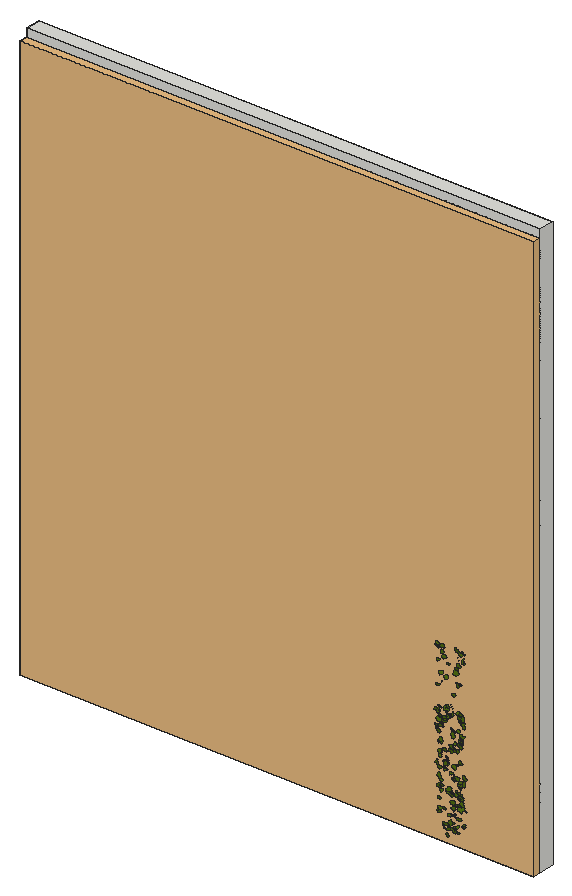
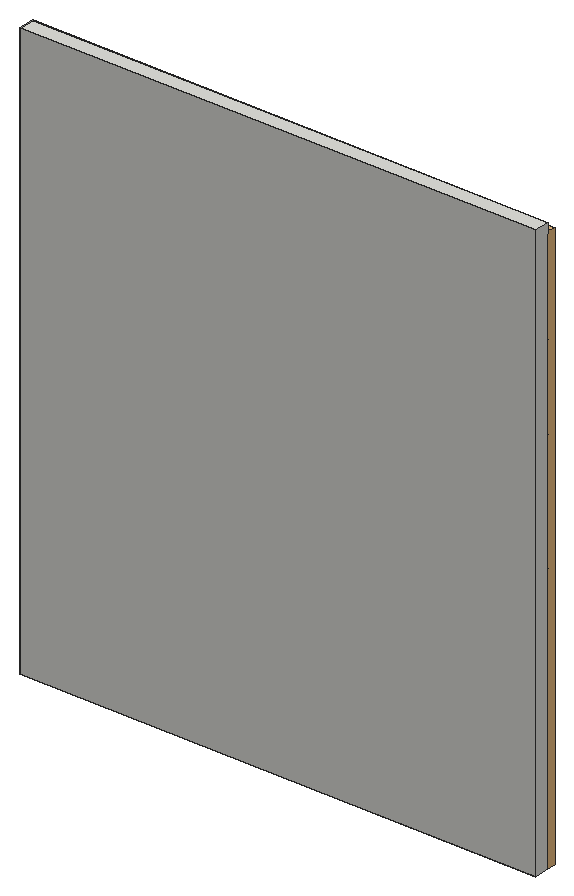
# SketchUp Ruby script. Lengths in inches.
U = 1.inch
M = Sketchup.active_model
def pt(a) = Geom::Point3d.new(a.map { |v| v * U })
def face(e, loops, mat)
  f = e.add_face(loops[0].map { |a| pt(a) })
  loops[1..].each { |l| e.add_face(l.map { |a| pt(a) }).erase! }
  f.material = f.back_material = mat if mat
  f
end
# faces: each face lists its corners as indices into pts; further lists are holes
def faces(e, pts, list, mat = nil) = list.each { |f| face(e, (f[0].is_a?(Array) ? f : [f]).map { |l| l.map { |i| pts[i] } }, mat) }
# xy, xz, yz: faces in a plane at the given z, y or x. An outline is a flat list of corners, or four numbers for a rectangle; further outlines are holes
def ring(l) = l.size == 4 ? [[l[0], l[1]], [l[2], l[1]], [l[2], l[3]], [l[0], l[3]]] : l.each_slice(2).to_a
def flat(e, list, mat, &to3) = list.each { |f| face(e, (f[0].is_a?(Array) ? f : [f]).map { |l| ring(l).map { |u, v| to3.(u, v) } }, mat) }
def xy(e, z, list, mat = nil) = flat(e, list, mat) { |x, y| [x, y, z] }
def xz(e, y, list, mat = nil) = flat(e, list, mat) { |x, z| [x, y, z] }
def yz(e, x, list, mat = nil) = flat(e, list, mat) { |y, z| [x, y, z] }
def lines(e, pts, list) = list.each { |a, b| e.add_line(pt(pts[a]), pt(pts[b])) }
# prism: a flat outline (further loops are holes) pulled along v
def prism(e, loops, v, mat = nil)
  f = face(e, loops, mat); d = Geom::Vector3d.new(v.map { |x| x * U })
  f.pushpull(f.normal.samedirection?(d) ? d.length : -d.length)
end
def box(e, o, s, mat = nil) = prism(e, [[o, [o[0] + s[0], o[1], o[2]], [o[0] + s[0], o[1] + s[1], o[2]], [o[0], o[1] + s[1], o[2]]]], [0, 0, s[2]], mat)
def at(x, y, z, deg = 0) = Geom::Transformation.translation(pt([x, y, z])) * Geom::Transformation.rotation(ORIGIN, Z_AXIS, deg.degrees)
def axes(o, x, y, z) = Geom::Transformation.new([*x, 0, *y, 0, *z, 0, *pt(o).to_a, 1])
def part(name) = M.definitions.add(name)
# library, detail: a bought-in or finely detailed component or shape, given as its bounding box
def library(name, o, s) = part(name).tap { |d| box(d.entities, o, s) }
def detail(e, o, s) = box(e.add_group.entities, o, s)
def put(e, d, t, mat = nil) = e.add_instance(d, t).tap { |i| i.material = mat if mat }
def group(e, t, mat = nil) = e.add_group.tap { |g| g.transformation = t; g.material = mat if mat }.entities
root = M.entities
M.materials.add("[Vegetation Blur 03]").color = [83, 114, 18]
c1 = library("Group\#9",[0,0,0],[130,2,144])
c2 = part("ivy")
xy(c2.entities,0,[[0.782,0,0.786,0,0.787,0.005,0.789,0.009,0.821,0.072,0.875,0.147,1.001,0.272,1.073,0.331,1.137,0.363,1.178,0.379,1.223,0.384,1.272,0.383,1.311,0.374,1.36,0.355,1.399,0.334,1.491,0.285,1.541,0.244,1.583,0.199,1.617,0.15,1.64,0.128,1.662,0.115,1.717,0.105,1.745,0.093,1.784,0.054,1.819,0.057,1.854,0.064,1.882,0.075,1.896,0.074,1.91,0.071,1.937,0.063,1.964,0.053,1.99,0.038,2.016,0.015,2.034,0.002,2.04,0,2.038,0.003,2.036,0.007,2.033,0.038,2.036,0.068,2.045,0.1,2.055,0.116,2.064,0.123,2.077,0.129,2.088,0.129,2.106,0.132,2.118,0.13,2.179,0.132,2.207,0.133,2.225,0.133,2.242,0.138,2.22,0.162,2.207,0.186,2.206,0.213,2.212,0.236,2.228,0.262,2.247,0.274,2.298,0.283,2.355,0.294,2.37,0.296,2.376,0.295,2.377,0.3,2.377,0.303,2.385,0.329,2.411,0.37,2.426,0.392,2.449,0.407,2.511,0.426,2.561,0.444,2.619,0.466,2.589,0.469,2.561,0.476,2.501,0.5,2.449,0.516,2.424,0.523,2.401,0.535,2.377,0.556,2.372,0.568,2.36,0.575,2.268,0.586,2.225,0.592,2.207,0.599,2.194,0.61,2.143,0.65,2.13,0.664,2.122,0.682,2.123,0.7,2.13,0.719,2.148,0.75,2.17,0.781,2.195,0.807,2.221,0.828,2.284,0.874,2.291,0.88,2.288,0.887,2.276,0.9,2.267,0.916,2.265,0.933,2.273,0.967,2.292,1.002,2.313,1.03,2.334,1.054,2.348,1.067,2.358,1.074,2.363,1.076,2.362,1.081,2.35,1.094,2.347,1.11,2.35,1.143,2.359,1.18,2.385,1.254,2.415,1.324,2.448,1.393,2.45,1.4,2.446,1.398,2.44,1.394,2.427,1.383,2.402,1.36,2.376,1.339,2.345,1.324,2.305,1.309,2.282,1.303,2.273,1.306,2.245,1.294,2.212,1.287,2.187,1.291,2.163,1.301,2.142,1.316,2.134,1.327,2.124,1.325,2.09,1.292,2.053,1.259,2.014,1.234,1.973,1.215,1.954,1.21,1.931,1.208,1.909,1.212,1.893,1.22,1.879,1.233,1.872,1.248,1.867,1.281,1.864,1.319,1.821,1.258,1.773,1.197,1.726,1.141,1.698,1.121,1.679,1.116,1.666,1.117,1.647,1.122,1.632,1.129,1.62,1.141,1.617,1.154,1.617,1.219,1.621,1.254,1.623,1.268,1.623,1.281,1.618,1.314,1.606,1.346,1.603,1.375,1.607,1.403,1.603,1.467,1.599,1.499,1.605,1.525,1.614,1.552,1.629,1.577,1.635,1.589,1.629,1.587,1.618,1.582,1.596,1.566,1.581,1.556,1.568,1.552,1.557,1.55,1.545,1.553,1.531,1.562,1.522,1.572,1.504,1.591,1.486,1.611,1.474,1.631,1.457,1.666,1.455,1.684,1.457,1.698,1.452,1.715,1.444,1.728,1.424,1.754,1.419,1.772,1.423,1.786,1.434,1.819,1.444,1.848,1.446,1.855,1.44,1.861,1.43,1.867,1.386,1.904,1.349,1.948,1.326,1.973,1.31,1.995,1.288,2.048,1.284,2.153,1.287,2.254,1.284,2.255,1.282,2.253,1.278,2.247,1.274,2.237,1.266,2.216,1.226,2.125,1.208,2.076,1.184,2.033,1.155,1.984,1.135,1.942,1.111,1.899,1.083,1.861,1.053,1.85,1.059,1.83,1.061,1.809,1.056,1.79,1.049,1.767,1.04,1.749,1.018,1.733,0.994,1.726,0.942,1.734,0.95,1.6875,0.944,1.645,0.932,1.608,0.911,1.585,0.881,1.58,0.854,1.582,0.828,1.588,0.785,1.618,0.773,1.625,0.775,1.614,0.779,1.598,0.796,1.502,0.818,1.402,0.861,1.283,0.882,1.224,0.894,1.174,0.892,1.148,0.886,1.123,0.881,1.107,0.872,1.099,0.849,1.094,0.818,1.092,0.789,1.098,0.762,1.107,0.753,1.113,0.721,1.139,0.698,1.163,0.678,1.194,0.665,1.224,0.628,1.28,0.612,1.312,0.606,1.327,0.606,1.314,0.599,1.282,0.594,1.267,0.581,1.256,0.544,1.245,0.512,1.244,0.473,1.249,0.444,1.256,0.382,1.288,0.339,1.306,0.324,1.316,0.317,1.324,0.309,1.326,0.27,1.314,0.227,1.313,0.185,1.3125,0.152,1.317,0.122,1.328,0.092,1.345,0.073,1.353,0.079,1.338,0.092,1.308,0.117,1.249,0.13,1.215,0.139,1.164,0.147,1.148,0.157,1.136,0.163,1.122,0.174,1.086,0.177,1.067,0.182,1.054,0.186,1.043,0.191,1.038,0.211,1.028,0.237,1.005,0.25,0.974,0.253,0.96,0.25,0.944,0.242,0.914,0.243,0.906,0.249,0.902,0.26,0.894,0.289,0.88,0.307,0.873,0.322,0.862,0.364,0.799,0.403,0.738,0.431,0.709,0.439,0.691,0.441,0.678,0.4375,0.66,0.428,0.645,0.394,0.623,0.303,0.594,0.255,0.581,0.214,0.577,0.179,0.573,0.173,0.568,0.175,0.561,0.167,0.55,0.141,0.523,0.113,0.503,0.077,0.49,0.045,0.486,0.026,0.485,0.019,0.486,0.011,0.483,0,0.471,0.014,0.467,0.044,0.455,0.058,0.447,0.07,0.438,0.097,0.411,0.125,0.394,0.158,0.377,0.174,0.366,0.182,0.359,0.185,0.361,0.242,0.331,0.253,0.316,0.258,0.303,0.262,0.283,0.274,0.278,0.308,0.274,0.341,0.252,0.366,0.226,0.366,0.222,0.37,0.22,0.38,0.221,0.395,0.221,0.425,0.216,0.45,0.207,0.465,0.192,0.473,0.178,0.484,0.15,0.489,0.116,0.483,0.089,0.468,0.058,0.45,0.035,0.435,0.018,0.429,0.011,0.434,0.012,0.438,0.014,0.469,0.019,0.542,0.016,0.581,0.015,0.612,0.027,0.68,0.055,0.696,0.057,0.712,0.052,0.73,0.045,0.741,0.036,0.766,0.014]])
put(root,c1,at(9,174,4))
g1 = group(root,at(4,176,4))
box(g1,[5,0,0],[130,4,146])
put(root,c2,axes([114.7,173.8,30.11],[0.07342,0.0201,-0.45241],[-0.55143,0.12193,-0.05876],[-0.05747,-1.14418,-0.01421]),"[Vegetation Blur 03]")
put(root,c2,axes([114.54,173.8,33.93],[0.13601,0.05917,-0.30855],[-0.37908,0.03752,-0.11017],[-0.00748,-0.82593,-0.02711]),"[Vegetation Blur 03]")
put(root,c2,axes([114.375,173.8,48.26],[0.33145,0.05992,-0.29685],[-0.36343,0.14447,-0.2657],[-0.03257,-1.00226,-0.05605]),"[Vegetation Blur 03]")
put(root,c2,axes([114.78,173.8,22.41],[0.27571,-0.25978,-0.33675],[-0.40528,0.18997,-0.24407],[-0.14812,-1.00337,0.04098]),"[Vegetation Blur 03]")
put(root,c2,axes([115.13,173.8,34.26],[0.12192,-0.00071,-0.41999],[-0.49465,0.29998,-0.09572],[-0.14193,-1.04612,-0.02717]),"[Vegetation Blur 03]")
put(root,c2,axes([115.16,173.8,34.28],[0.14174,-0.20689,-0.42841],[-0.51411,0.25268,-0.13249],[-0.14609,-1.08996,0.0506]),"[Vegetation Blur 03]")
put(root,c2,axes([114.39,173.8,39.43],[0.38883,0.03177,-0.00541],[-0.00902,0.12865,-0.31342],[0.01417,-0.78985,-0.05127]),"[Vegetation Blur 03]")
put(root,c2,axes([114.64,173.8,45.22],[0.29737,0.00668,-0.03254],[-0.03987,-0.00069,-0.24271],[0.00326,-0.6174,-0.00008]),"[Vegetation Blur 03]")
put(root,c2,axes([114.17,173.8,48.53],[0.22945,0.18892,0.3925],[0.48869,-0.02142,-0.18866],[0.02999,-1.09631,0.07132]),"[Vegetation Blur 03]")
put(root,c2,axes([115.12,173.8,34.72],[0.32489,0.11128,-0.34401],[-0.42351,0.17483,-0.25752],[-0.03505,-1.08109,-0.07706]),"[Vegetation Blur 03]")
put(root,c2,axes([114.58,173.8,29.73],[0.57169,-0.21875,-0.18427],[-0.21197,0.1873,-0.473],[-0.13171,-1.2509,-0.0386]),"[Vegetation Blur 03]")
put(root,c2,axes([115.09,173.8,14.08],[0.26898,-0.00531,-0.22272],[-0.27011,0.10743,-0.21769],[-0.03898,-0.78115,-0.02842]),"[Vegetation Blur 03]")
put(root,c2,axes([115.41,173.8,19.51],[0.26861,-0.16753,-0.42435],[-0.51691,0.14174,-0.22674],[-0.09889,-1.19591,0.03257]),"[Vegetation Blur 03]")
put(root,c2,axes([114.76,173.8,32.02],[0.48108,0.0091,-0.09014],[-0.10924,-0.11608,-0.39016],[0.0169,-1.00907,0.04407]),"[Vegetation Blur 03]")
put(root,c2,axes([115.22,173.8,11.125],[0.44397,0.1395,-0.34863],[-0.43136,0.05055,-0.3627],[0.03168,-1.26682,-0.05286]),"[Vegetation Blur 03]")
put(root,c2,axes([115.18,173.8,16.72],[0.30297,0.01543,-0.16149],[-0.19571,0.1367,-0.2425],[-0.03016,-0.73198,-0.04869]),"[Vegetation Blur 03]")
put(root,c2,axes([115.17,173.8,11.875],[0.36198,-0.00364,-0.10329],[-0.12566,-0.10485,-0.29275],[0.01516,-0.7821,0.03972]),"[Vegetation Blur 03]")
put(root,c2,axes([115.8125,173.8,40.52],[0.10541,0.02404,-0.33372],[-0.3979,0.2077,-0.08136],[-0.09494,-0.84377,-0.02954]),"[Vegetation Blur 03]")
put(root,c2,axes([114.77,173.8,24.11],[0.22933,0.01454,0.32661],[0.40022,0.004,-0.18721],[0.0052,-0.94915,0.00421]),"[Vegetation Blur 03]")
put(root,c2,axes([114.95,173.8,21.01],[0.4011,-0.07198,0.04538],[0.05521,-0.01426,-0.32859],[-0.0356,-0.83315,0.0017]),"[Vegetation Blur 03]")
put(root,c2,axes([115.11,173.8,32.88],[0.3582,-0.18702,-0.03708],[-0.03384,0.10347,-0.29982],[-0.09581,-0.73577,-0.03274]),"[Vegetation Blur 03]")
put(root,c2,axes([114.42,173.8,16.34],[0.50593,-0.03643,0.3437],[0.41936,0.17969,-0.40818],[0.0424,-1.34262,-0.06395]),"[Vegetation Blur 03]")
put(root,c2,axes([115.83,173.8,27.52],[0.12968,-0.11784,-0.31424],[-0.38451,0.09135,-0.11108],[-0.06065,-0.83104,0.03235]),"[Vegetation Blur 03]")
put(root,c2,axes([115.125,173.8,23.08],[0.14273,0.06127,0.20808],[0.25666,-0.04237,-0.11531],[-0.00355,-0.59977,0.0294]),"[Vegetation Blur 03]")
put(root,c2,axes([114.82,173.8,26.49],[0.3729,0.07352,0.23123],[0.28448,-0.01242,-0.30497],[0.02479,-0.96364,0.02157]),"[Vegetation Blur 03]")
put(root,c2,axes([115.39,173.8,30.48],[0.49872,0.09657,-0.2358],[-0.29251,0.12066,-0.4043],[0.0109,-1.17989,-0.06065]),"[Vegetation Blur 03]")
put(root,c2,axes([115.37,173.8,30.86],[0.33145,-0.08577,-0.02014],[-0.01771,0.11215,-0.26935],[-0.04508,-0.6747,-0.04221]),"[Vegetation Blur 03]")
put(root,c2,axes([114.73,173.8,31.82],[0.38163,0.10723,0.44815],[0.5511,-0.01709,-0.31195],[0.0229,-1.37595,0.0388]),"[Vegetation Blur 03]")
put(root,c2,axes([115.05,173.8,42.07],[0.21319,0.1755,0.40106],[0.49372,-0.23014,-0.15897],[-0.07069,-1.078,0.09923]),"[Vegetation Blur 03]")
put(root,c2,axes([115.49,173.8,15.84],[0.32221,-0.0387,0.02273],[0.02664,-0.04287,-0.26295],[-0.0205,-0.66413,0.01565]),"[Vegetation Blur 03]")
put(root,c2,axes([115.57,173.8,46.77],[0.07701,-0.01607,0.28736],[0.35217,-0.0014,-0.06288],[-0.00233,-0.74167,-0.00611]),"[Vegetation Blur 03]")
put(root,c2,axes([115.125,173.8,17.75],[0.25598,0.2014,0.48378],[0.59803,0.04143,-0.21349],[0.05748,-1.32803,0.06671]),"[Vegetation Blur 03]")
put(root,c2,axes([115.4375,173.8,48.13],[0.23882,-0.04134,0.29544],[0.36225,0.06442,-0.19363],[0.01513,-0.89011,-0.02773]),"[Vegetation Blur 03]")
put(root,c2,axes([116.13,173.8,7.89],[0.29522,-0.08617,-0.18688],[-0.21829,0.16177,-0.24143],[-0.08083,-0.75161,-0.03054]),"[Vegetation Blur 03]")
put(root,c2,axes([115.88,173.8,31.86],[0.50551,0.02715,-0.04471],[-0.05585,0.1053,-0.41049],[0.00753,-1.04102,-0.04269]),"[Vegetation Blur 03]")
put(root,c2,axes([116.46,173.8,11.91],[0.2455,0.02361,-0.20397],[-0.24867,0.10235,-0.19749],[-0.02754,-0.71362,-0.03507]),"[Vegetation Blur 03]")
put(root,c2,axes([116.5,173.8,22.6],[0.23892,0.03876,-0.2007],[-0.24369,0.14566,-0.1888],[-0.038,-0.69034,-0.0511]),"[Vegetation Blur 03]")
put(root,c2,axes([116.77,173.8,25.42],[0.22065,0.07279,-0.34055],[-0.41864,0.06201,-0.17859],[-0.01021,-0.96933,-0.037]),"[Vegetation Blur 03]")
put(root,c2,axes([115.95,173.8,45.74],[0.16739,0.00231,0.3142],[0.38437,0.04772,-0.13645],[0.02172,-0.86254,-0.00671]),"[Vegetation Blur 03]")
put(root,c2,axes([116.51,173.8,21.24],[0.33471,0.047,-0.24757],[-0.30145,0.17573,-0.26622],[-0.0408,-0.91277,-0.064]),"[Vegetation Blur 03]")
put(root,c2,axes([116.29,173.8,20.37],[0.12441,0.10653,0.22366],[0.27873,-0.02631,-0.1013],[0.00957,-0.61876,0.04281]),"[Vegetation Blur 03]")
put(root,c2,axes([117.41,173.8,23.6],[0.10808,0.0782,-0.51354],[-0.62715,0.14615,-0.08441],[-0.06373,-1.30565,-0.04021]),"[Vegetation Blur 03]")
put(root,c2,axes([116.26,173.8,32.03],[0.20968,0.01131,0.23173],[0.28004,-0.12895,-0.16779],[-0.0472,-0.71481,0.03394]),"[Vegetation Blur 03]")
put(root,c2,axes([116.51,173.8,22.875],[0.56655,-0.0115,-0.27779],[-0.34007,0.04247,-0.46224],[-0.01542,-1.35941,-0.01209]),"[Vegetation Blur 03]")
put(root,c2,axes([116.84,173.8,34.89],[0.41729,-0.27977,-0.39423],[-0.44817,0.37379,-0.3577],[-0.22574,-1.25924,-0.01859]),"[Vegetation Blur 03]")
put(root,c2,axes([116.05,173.8,8.41],[0.53014,0.02962,0.10212],[0.12282,0.12551,-0.4304],[0.02794,-1.11386,-0.04578]),"[Vegetation Blur 03]")
put(root,c2,axes([117.2,173.8,23.35],[0.21226,-0.08156,-0.39258],[-0.47103,0.20087,-0.17619],[-0.10528,-1.06312,-0.00317]),"[Vegetation Blur 03]")
put(root,c2,axes([116.26,173.8,31.98],[0.16066,-0.07376,0.37357],[0.45903,0.04715,-0.13002],[0.00982,-0.99714,-0.03378]),"[Vegetation Blur 03]")
put(root,c2,axes([116.93,173.8,35.1],[0.38856,-0.00058,-0.29483],[-0.35992,-0.09405,-0.31593],[0.03091,-1.0877,0.02748]),"[Vegetation Blur 03]")
put(root,c2,axes([116.41,173.8,41.5],[0.24024,0.06291,0.29442],[0.3619,-0.06648,-0.19446],[-0.01006,-0.88941,0.03536]),"[Vegetation Blur 03]")
put(root,c2,axes([116.96,173.8,33.74],[0.55985,-0.09656,-0.30764],[-0.35518,0.35678,-0.44814],[-0.13469,-1.34226,-0.09699]),"[Vegetation Blur 03]")
put(root,c2,axes([117.27,173.8,6.25],[0.22842,-0.06235,-0.19773],[-0.23665,0.11144,-0.18763],[-0.06007,-0.67607,-0.01269]),"[Vegetation Blur 03]")
put(root,c2,axes([117.18,173.8,35.52],[0.31144,-0.00755,-0.1936],[-0.23722,0.00118,-0.25419],[-0.00327,-0.80561,0.00144]),"[Vegetation Blur 03]")
put(root,c2,axes([117.15,173.8,44.96],[0.30877,0.02964,-0.06253],[-0.07793,0.09874,-0.24894],[0.00225,-0.64717,-0.04084]),"[Vegetation Blur 03]")
put(root,c2,axes([118.29,173.8,7.86],[0.10967,0.16764,-0.53959],[-0.66571,-0.0227,-0.09123],[0.02429,-1.37893,-0.0641]),"[Vegetation Blur 03]")
put(root,c2,axes([116.76,173.8,15.87],[0.43423,0.11965,0.28912],[0.35873,-0.10053,-0.35232],[0.01383,-1.14881,0.06094]),"[Vegetation Blur 03]")
put(root,c2,axes([116.99,173.8,32.98],[0.34318,0.09184,0.26358],[0.326,-0.10859,-0.27677],[-0.00403,-0.96364,0.05631]),"[Vegetation Blur 03]")
put(root,c2,axes([117.25,173.8,10.47],[0.24944,0.02336,0.19362],[0.23616,0.05082,-0.20362],[0.02524,-0.70655,-0.00824]),"[Vegetation Blur 03]")
put(root,c2,axes([117.93,173.8,15.9],[0.17883,0.01791,-0.19414],[-0.23754,0.05276,-0.14498],[-0.01529,-0.61012,-0.01823]),"[Vegetation Blur 03]")
put(root,c2,axes([116.83,173.8,15.91],[0.34678,0.03788,0.46084],[0.56412,0.05104,-0.28341],[0.03077,-1.36263,0.00219]),"[Vegetation Blur 03]")
put(root,c2,axes([118.625,173.8,19.15],[0.17288,0.13727,-0.46997],[-0.57483,0.20036,-0.13164],[-0.0749,-1.22089,-0.07445]),"[Vegetation Blur 03]")
put(root,c2,axes([117.64,173.8,26.55],[0.40772,-0.01716,0.08723],[0.10718,0.04684,-0.33224],[-0.00228,-0.8661,-0.01969]),"[Vegetation Blur 03]")
put(root,c2,axes([118.08,173.8,20.62],[0.28445,-0.01133,-0.1134],[-0.139,-0.04223,-0.23156],[0.00407,-0.65007,0.01702]),"[Vegetation Blur 03]")
put(root,c2,axes([118.01,173.8,35.88],[0.40706,-0.21039,-0.21028],[-0.21941,0.3311,-0.33502],[-0.1694,-0.93442,-0.07136]),"[Vegetation Blur 03]")
put(root,c2,axes([117.52,173.8,8.53],[0.18345,-0.01602,0.41607],[0.50825,-0.08298,-0.14976],[-0.04057,-1.11184,0.00518]),"[Vegetation Blur 03]")
put(root,c2,axes([117.6,173.8,25.625],[0.48848,-0.12647,0.08295],[0.10536,0.05262,-0.40062],[-0.05484,-1.02537,-0.03079]),"[Vegetation Blur 03]")
put(root,c2,axes([118.01,173.8,15.94],[0.464,-0.18688,-0.09777],[-0.10719,0.14954,-0.38378],[-0.10541,-0.97473,-0.04013]),"[Vegetation Blur 03]")
put(root,c2,axes([118.87,173.8,34.38],[0.12813,-0.15006,-0.36786],[-0.44192,0.20151,-0.11546],[-0.11482,-0.94298,0.03387]),"[Vegetation Blur 03]")
put(root,c2,axes([118.32,173.8,11.03],[0.53027,0.09687,-0.32245],[-0.39653,0.24084,-0.42296],[-0.03295,-1.33931,-0.09938]),"[Vegetation Blur 03]")
put(root,c2,axes([117.9375,173.8,30.54],[0.61753,-0.18671,-0.12394],[-0.12621,0.33022,-0.49708],[-0.12397,-1.26626,-0.11135]),"[Vegetation Blur 03]")
put(root,c2,axes([118.89,173.8,20.17],[0.24952,-0.09563,-0.45788],[-0.54485,0.27669,-0.20686],[-0.14163,-1.23287,-0.01091]),"[Vegetation Blur 03]")
put(root,c2,axes([118.68,173.8,9.23],[0.30579,0.15468,-0.23311],[-0.2938,0.07258,-0.24913],[0.03027,-0.858,-0.0631]),"[Vegetation Blur 03]")
put(root,c2,axes([119.15,173.8,29.98],[0.21628,-0.19716,-0.4852],[-0.59473,0.13393,-0.18514],[-0.09444,-1.29492,0.05473]),"[Vegetation Blur 03]")
put(root,c2,axes([117.97,173.8,13.84],[0.46672,-0.03992,0.15461],[0.18977,0.01161,-0.3811],[-0.01585,-1.03645,-0.01022]),"[Vegetation Blur 03]")
put(root,c2,axes([118.35,173.8,38.17],[0.33638,0.01493,0.11781],[0.14294,0.07701,-0.27338],[0.02139,-0.74929,-0.02575]),"[Vegetation Blur 03]")
put(root,c2,axes([118.21,173.8,12.24],[0.25126,-0.00237,0.3092],[0.37875,0.02524,-0.20497],[0.00958,-0.93516,-0.00632]),"[Vegetation Blur 03]")
put(root,c2,axes([118.5625,173.8,26.54],[0.44154,-0.10792,-0.13293],[-0.15664,0.11844,-0.36167],[-0.06888,-0.96117,-0.02964]),"[Vegetation Blur 03]")
put(root,c2,axes([118.58,173.8,26.13],[0.39751,-0.09835,-0.09675],[-0.112,0.11608,-0.32505],[-0.0616,-0.84567,-0.03337]),"[Vegetation Blur 03]")
put(root,c2,axes([119.46,173.8,22.44],[0.06394,-0.03491,-0.38067],[-0.46672,-0.01334,-0.05203],[0.00412,-0.96871,0.01444]),"[Vegetation Blur 03]")
put(root,c2,axes([118.11,173.8,7.51],[0.43162,0.02667,0.37239],[0.45622,0.01814,-0.35241],[0.01531,-1.29236,0.00274]),"[Vegetation Blur 03]")
put(root,c2,axes([118.76,173.8,11.9],[0.51252,-0.27009,-0.18144],[-0.18784,0.30748,-0.42542],[-0.17711,-1.10772,-0.07385]),"[Vegetation Blur 03]")
put(root,c2,axes([118.82,173.8,8.04],[0.4822,-0.17189,-0.16775],[-0.19534,0.15084,-0.39833],[-0.10519,-1.06807,-0.02926]),"[Vegetation Blur 03]")
put(root,c2,axes([118.97,173.8,27.02],[0.11399,0.08931,0.26369],[0.32563,0.00233,-0.09389],[0.01551,-0.70503,0.03309]),"[Vegetation Blur 03]")
put(root,c2,axes([119.8,173.8,13.51],[0.24902,0.09318,-0.40988],[-0.50306,0.12516,-0.1991],[-0.03467,-1.14673,-0.05504]),"[Vegetation Blur 03]")
put(root,c2,axes([118.81,173.8,42.76],[0.09049,0.02962,0.47011],[0.57571,0.04471,-0.07426],[0.0237,-1.19903,0.00884]),"[Vegetation Blur 03]")
put(root,c2,axes([119.92,173.8,46.97],[0.14161,0.02749,-0.37414],[-0.43235,0.33737,-0.1051],[-0.153,-0.92792,-0.0493]),"[Vegetation Blur 03]")
put(root,c2,axes([119.18,173.8,49.125],[0.51011,-0.11701,-0.13612],[-0.15838,0.15628,-0.41647],[-0.07724,-1.09327,-0.04497]),"[Vegetation Blur 03]")
put(root,c2,axes([119.6875,173.8,41.34],[0.31562,-0.0779,-0.30416],[-0.3657,0.1532,-0.25894],[-0.08116,-0.99323,-0.01608]),"[Vegetation Blur 03]")
put(root,c2,axes([119.29,173.8,7.54],[0.43132,0.00683,-0.12215],[-0.14822,0.15148,-0.34728],[-0.02104,-0.9272,-0.05763]),"[Vegetation Blur 03]")
put(root,c2,axes([118.98,173.8,22.54],[0.54712,0.06533,0.00829],[0.00324,0.23778,-0.43729],[0.03318,-1.10066,-0.09398]),"[Vegetation Blur 03]")
put(root,c2,axes([118.9375,173.8,26.03],[0.51598,-0.04836,0.08245],[0.10256,0.07999,-0.4201],[-0.01553,-1.07898,-0.03484]),"[Vegetation Blur 03]")
put(root,c2,axes([119.17,173.8,44.5],[0.35213,-0.1038,0.09821],[0.12718,0.11373,-0.28482],[-0.02917,-0.75727,-0.05624]),"[Vegetation Blur 03]")
put(root,c2,axes([119.01,173.8,15.54],[0.19537,0.05525,0.44525],[0.54604,-0.05051,-0.1586],[-0.01409,-1.19141,0.02737]),"[Vegetation Blur 03]")
put(root,c2,axes([119.39,173.8,19.97],[0.45876,-0.06676,-0.02085],[-0.02631,-0.02088,-0.37522],[-0.03182,-0.94526,0.00976]),"[Vegetation Blur 03]")
put(root,c2,axes([119.49,173.8,8.47],[0.21181,0.06558,0.16158],[0.19963,-0.12494,-0.16633],[-0.01894,-0.58339,0.05378]),"[Vegetation Blur 03]")
put(root,c2,axes([120.14,173.8,45.78],[0.26725,0.04128,-0.32232],[-0.39537,0.00799,-0.21819],[0.00802,-0.98126,-0.01534]),"[Vegetation Blur 03]")
put(root,c2,axes([119.53,173.8,34.23],[0.21448,0.07418,0.20841],[0.25788,-0.06923,-0.1729],[-0.00284,-0.68276,0.04017]),"[Vegetation Blur 03]")
put(root,c2,axes([120.35,173.8,17.58],[0.21131,0.04206,-0.34485],[-0.41038,0.25638,-0.16258],[-0.10272,-0.93777,-0.05992]),"[Vegetation Blur 03]")
put(root,c2,axes([119.59,173.8,30.15],[0.18344,0.08958,0.24161],[0.29922,-0.05038,-0.14838],[0.0019,-0.7149,0.04073]),"[Vegetation Blur 03]")
put(root,c2,axes([119.67,173.8,10.68],[0.44484,-0.01751,0.04002],[0.04967,0.10203,-0.36079],[-0.00297,-0.91526,-0.04099]),"[Vegetation Blur 03]")
put(root,c2,axes([119.73,173.8,16.36],[0.36338,-0.06137,0.0857],[0.10665,0.03955,-0.29676],[-0.02326,-0.77736,-0.02186]),"[Vegetation Blur 03]")
put(root,c2,axes([119.78,173.8,27.66],[0.62172,-0.07982,-0.18766],[-0.22411,0.16779,-0.50577],[-0.06444,-1.35373,-0.05162]),"[Vegetation Blur 03]")
put(root,c2,axes([120.27,173.8,32.71],[0.25042,-0.03463,-0.18206],[-0.21423,0.16131,-0.2011],[-0.06442,-0.671,-0.03895]),"[Vegetation Blur 03]")
put(root,c2,axes([120.72,173.8,41.26],[0.07231,0.11382,-0.30015],[-0.37128,0.06711,-0.05557],[-0.02172,-0.76837,-0.04931]),"[Vegetation Blur 03]")
put(root,c2,axes([119.95,173.8,33.65],[0.43667,-0.00599,-0.05285],[-0.0643,0.07555,-0.35518],[-0.00825,-0.90526,-0.02929]),"[Vegetation Blur 03]")
put(root,c2,axes([120.36,173.8,28.3],[0.37381,-0.01776,-0.27785],[-0.3272,0.26974,-0.29592],[-0.09444,-1.00486,-0.07453]),"[Vegetation Blur 03]")
put(root,c2,axes([120.05,173.8,13.36],[0.12453,-0.12682,0.21988],[0.27637,0.0612,-0.0987],[0.00185,-0.60769,-0.05583]),"[Vegetation Blur 03]")
put(root,c2,axes([120.62,173.8,23.83],[0.24891,0.01709,-0.28911],[-0.35411,0.04401,-0.20266],[-0.01273,-0.88984,-0.01558]),"[Vegetation Blur 03]")
put(root,c2,axes([121.07,173.8,19.13],[0.07751,-0.08641,-0.39879],[-0.48715,0.10409,-0.06661],[-0.05668,-1.01274,0.02718]),"[Vegetation Blur 03]")
put(root,c2,axes([120.42,173.8,28.97],[0.45681,-0.21004,-0.23078],[-0.27305,0.15298,-0.3819],[-0.12578,-1.09491,-0.00909]),"[Vegetation Blur 03]")
put(root,c2,axes([119.99,173.8,15.1875],[0.0827,0.01826,0.45445],[0.55686,-0.01784,-0.06738],[-0.00727,-1.15829,0.0082]),"[Vegetation Blur 03]")
put(root,c2,axes([119.875,173.8,18.28],[0.50405,-0.0121,0.1413],[0.17315,0.00073,-0.4114],[-0.00545,-1.09673,-0.00183]),"[Vegetation Blur 03]")
put(root,c2,axes([120.11,173.8,34.17],[0.30561,-0.04373,0.17256],[0.21196,0.11676,-0.24539],[0.01507,-0.75575,-0.0479]),"[Vegetation Blur 03]")
put(root,c2,axes([120.27,173.8,48.17],[0.38022,-0.03036,0.06928],[0.08439,-0.02832,-0.31043],[-0.01739,-0.80118,0.00835]),"[Vegetation Blur 03]")
put(root,c2,axes([121.29,173.8,28.72],[0.06632,-0.08264,-0.34848],[-0.42857,0.02082,-0.0551],[-0.0162,-0.88896,0.0311]),"[Vegetation Blur 03]")
put(root,c2,axes([119.89,173.8,14.95],[0.37722,-0.01424,0.37521],[0.45787,0.12358,-0.30587],[0.04206,-1.2175,-0.03543]),"[Vegetation Blur 03]")
put(root,c2,axes([119.92,173.8,13.12],[0.61342,0.08443,0.16311],[0.20359,-0.16924,-0.49623],[0.01316,-1.31678,0.07424]),"[Vegetation Blur 03]")
put(root,c2,axes([121.44,173.8,34.22],[0.15478,-0.07462,-0.45486],[-0.55676,0.07347,-0.12809],[-0.04416,-1.18802,0.02065]),"[Vegetation Blur 03]")
put(root,c2,axes([121.05,173.8,48.67],[0.32569,0.04627,-0.29452],[-0.35796,0.18221,-0.25916],[-0.05099,-0.98359,-0.06186]),"[Vegetation Blur 03]")
put(root,c2,axes([120.7,173.8,29.87],[0.44969,-0.01244,-0.10758],[-0.13185,-0.00591,-0.36702],[-0.00499,-0.96429,0.00364]),"[Vegetation Blur 03]")
put(root,c2,axes([121.65,173.8,47.54],[0.07293,-0.28065,-0.423],[-0.50755,0.30955,-0.09059],[-0.17213,-1.03162,0.0879]),"[Vegetation Blur 03]")
put(root,c2,axes([120.44,173.8,13.63],[0.13579,0.06981,0.42324],[0.51409,-0.17958,-0.1052],[-0.07611,-1.08841,0.0445]),"[Vegetation Blur 03]")
put(root,c2,axes([121.52,173.8,46.51],[0.10604,0.023,-0.23018],[-0.28135,0.05824,-0.08542],[-0.02259,-0.61729,-0.01663]),"[Vegetation Blur 03]")
put(root,c2,axes([121.62,173.8,32.93],[0.29092,-0.24551,-0.40873],[-0.49509,0.19114,-0.25278],[-0.14116,-1.1764,0.04423]),"[Vegetation Blur 03]")
put(root,c2,axes([121.78,173.8,19.91],[0.26701,-0.30376,-0.4486],[-0.53833,0.27065,-0.24226],[-0.1847,-1.22801,0.05757]),"[Vegetation Blur 03]")
put(root,c2,axes([122.04,173.8,12.76],[0.09506,0.21771,-0.46057],[-0.55663,0.32363,-0.05246],[-0.14082,-1.13231,-0.10355]),"[Vegetation Blur 03]")
put(root,c2,axes([121.67,173.8,20.89],[0.30205,-0.06223,-0.36549],[-0.44449,0.11303,-0.2477],[-0.06243,-1.1058,-0.00475]),"[Vegetation Blur 03]")
put(root,c2,axes([121.1,173.8,9.14],[0.28399,-0.06546,0.07539],[0.09562,0.06624,-0.23087],[-0.02006,-0.61097,-0.03311]),"[Vegetation Blur 03]")
put(root,c2,axes([121.03,173.8,9.02],[0.18546,0.05213,0.26962],[0.33131,-0.03649,-0.15069],[-0.00311,-0.77875,0.02511]),"[Vegetation Blur 03]")
